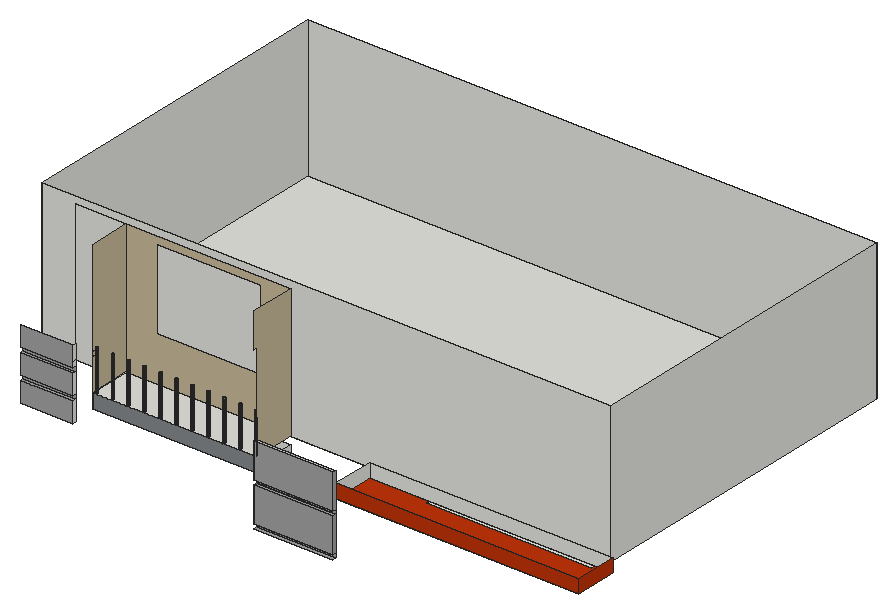
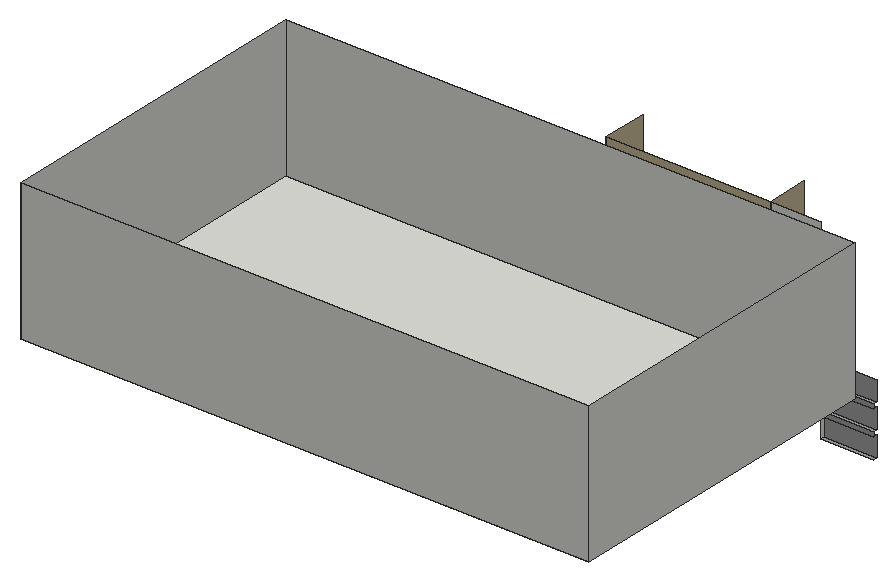
# SketchUp Ruby script. Lengths in inches.
U = 1.inch
M = Sketchup.active_model
def pt(a) = Geom::Point3d.new(a.map { |v| v * U })
def face(e, loops, mat)
  f = e.add_face(loops[0].map { |a| pt(a) })
  loops[1..].each { |l| e.add_face(l.map { |a| pt(a) }).erase! }
  f.material = f.back_material = mat if mat
  f
end
# faces: each face lists its corners as indices into pts; further lists are holes
def faces(e, pts, list, mat = nil) = list.each { |f| face(e, (f[0].is_a?(Array) ? f : [f]).map { |l| l.map { |i| pts[i] } }, mat) }
# xy, xz, yz: faces in a plane at the given z, y or x. An outline is a flat list of corners, or four numbers for a rectangle; further outlines are holes
def ring(l) = l.size == 4 ? [[l[0], l[1]], [l[2], l[1]], [l[2], l[3]], [l[0], l[3]]] : l.each_slice(2).to_a
def flat(e, list, mat, &to3) = list.each { |f| face(e, (f[0].is_a?(Array) ? f : [f]).map { |l| ring(l).map { |u, v| to3.(u, v) } }, mat) }
def xy(e, z, list, mat = nil) = flat(e, list, mat) { |x, y| [x, y, z] }
def xz(e, y, list, mat = nil) = flat(e, list, mat) { |x, z| [x, y, z] }
def yz(e, x, list, mat = nil) = flat(e, list, mat) { |y, z| [x, y, z] }
def lines(e, pts, list) = list.each { |a, b| e.add_line(pt(pts[a]), pt(pts[b])) }
# prism: a flat outline (further loops are holes) pulled along v
def prism(e, loops, v, mat = nil)
  f = face(e, loops, mat); d = Geom::Vector3d.new(v.map { |x| x * U })
  f.pushpull(f.normal.samedirection?(d) ? d.length : -d.length)
end
def box(e, o, s, mat = nil) = prism(e, [[o, [o[0] + s[0], o[1], o[2]], [o[0] + s[0], o[1] + s[1], o[2]], [o[0], o[1] + s[1], o[2]]]], [0, 0, s[2]], mat)
def at(x, y, z, deg = 0) = Geom::Transformation.translation(pt([x, y, z])) * Geom::Transformation.rotation(ORIGIN, Z_AXIS, deg.degrees)
def axes(o, x, y, z) = Geom::Transformation.new([*x, 0, *y, 0, *z, 0, *pt(o).to_a, 1])
def part(name) = M.definitions.add(name)
# library, detail: a bought-in or finely detailed component or shape, given as its bounding box
def library(name, o, s) = part(name).tap { |d| box(d.entities, o, s) }
def detail(e, o, s) = box(e.add_group.entities, o, s)
def put(e, d, t, mat = nil) = e.add_instance(d, t).tap { |i| i.material = mat if mat }
def group(e, t, mat = nil) = e.add_group.tap { |g| g.transformation = t; g.material = mat if mat }.entities
root = M.entities
M.materials.add("[0133_Gray]").color = [128, 128, 128]
M.materials.add("[Blacktop New]").color = [30, 30, 30]
M.materials.add("[Blacktop Old 01]").color = [132, 136, 139]
M.materials.add("[Marble Carrara Gold Floor Tile]").color = [225, 223, 217]
M.materials.add("[Modern Siding]1").color = [191, 52, 9]
M.materials.add("[Pavers Flagstone Gray]").color = [162, 162, 162]
M.materials.add("[Quartz Light Brown]").color = [199, 184, 152]
xy(root,432.5,[[229.62,0,297.58,3]],"[Pavers Flagstone Gray]")
xy(root,432.57,[[0,36,45.0625,39]],"[Pavers Flagstone Gray]")
xy(root,436.12,[[229.62,0,297.58,3]],"[Pavers Flagstone Gray]")
xy(root,449.9375,[[0,36,45.0625,39]],"[Pavers Flagstone Gray]")
xy(root,454.01,[[0,36,45.0625,39]],"[Pavers Flagstone Gray]")
xy(root,464.74,[[127.42,36,161.55,39],[163.99,36,195.67,39]],"[Blacktop New]")
xy(root,466,[[229.62,0,297.58,3]],"[Pavers Flagstone Gray]")
xy(root,467.74,[[124.42,36,198.67,39]],"[Blacktop New]")
xy(root,469.62,[[229.62,0,297.58,3]],"[Pavers Flagstone Gray]")
xy(root,471.375,[[0,36,45.0625,39]],"[Pavers Flagstone Gray]")
xy(root,472.125,[[355.33,36,420.06,39],[424.01,36,484.79,39]],"[Blacktop New]")
xy(root,473.6875,[[88.53,3,229.62,39]],"[Blacktop Old 01]")
xy(root,475.45,[[0,36,45.0625,39]],"[Pavers Flagstone Gray]")
xy(root,478.125,[[349.33,36,490.79,39]])
xy(root,478.125,[[297.58,3,297.58,39,349.33,39,349.33,36,490.79,36,490.79,39,506.625,39,506.625,3]],"[Modern Siding]1")
xy(root,480,[[9,48,497.625,333.4375]])
xy(root,486.23,[[[88.53,3,229.62,39],[104.73,3.35,104.5,3.39,104.3,3.49,104.13,3.65,104,3.84,103.93,4.05,103.92,4.28,103.97,4.51,104.07,4.71,104.22,4.88,104.41,5.01,104.63,5.08,104.86,5.09,105.08,5.04,105.28,4.94,105.45,4.79,105.58,4.6,105.65,4.38,105.66,4.15,105.62,3.93,105.51,3.73,105.36,3.55,105.17,3.43,104.95,3.36],[118.41,3.35,118.19,3.39,117.99,3.49,117.82,3.65,117.69,3.84,117.62,4.05,117.61,4.28,117.65,4.51,117.76,4.71,117.91,4.88,118.1,5.01,118.32,5.08,118.54,5.09,118.77,5.04,118.97,4.94,119.14,4.79,119.27,4.6,119.34,4.38,119.35,4.15,119.31,3.93,119.2,3.73,119.05,3.55,118.86,3.43,118.64,3.36],[132.1,3.35,131.88,3.39,131.67,3.49,131.5,3.65,131.38,3.84,131.31,4.05,131.29,4.28,131.34,4.51,131.44,4.71,131.6,4.88,131.79,5.01,132,5.08,132.23,5.09,132.46,5.04,132.66,4.94,132.83,4.79,132.95,4.6,133.03,4.38,133.04,4.15,132.99,3.93,132.89,3.73,132.74,3.55,132.55,3.43,132.33,3.36],[145.79,3.35,145.57,3.39,145.36,3.49,145.19,3.65,145.07,3.84,144.99,4.05,144.98,4.28,145.03,4.51,145.13,4.71,145.28,4.88,145.47,5.01,145.69,5.08,145.92,5.09,146.14,5.04,146.35,4.94,146.52,4.79,146.64,4.6,146.71,4.38,146.73,4.15,146.68,3.93,146.58,3.73,146.43,3.55,146.23,3.43,146.02,3.36],[159.48,3.35,159.25,3.39,159.05,3.49,158.88,3.65,158.75,3.84,158.68,4.05,158.67,4.28,158.72,4.51,158.82,4.71,158.97,4.88,159.16,5.01,159.38,5.08,159.61,5.09,159.83,5.04,160.03,4.94,160.2,4.79,160.33,4.6,160.4,4.38,160.41,4.15,160.37,3.93,160.26,3.73,160.11,3.55,159.92,3.43,159.7,3.36],[173.16,3.35,172.94,3.39,172.74,3.49,172.57,3.65,172.44,3.84,172.37,4.05,172.36,4.28,172.4,4.51,172.51,4.71,172.66,4.88,172.85,5.01,173.07,5.08,173.29,5.09,173.52,5.04,173.72,4.94,173.89,4.79,174.02,4.6,174.09,4.38,174.1,4.15,174.06,3.93,173.95,3.73,173.8,3.55,173.61,3.43,173.39,3.36],[91.04,3.35,90.82,3.39,90.61,3.49,90.44,3.65,90.32,3.84,90.24,4.05,90.23,4.28,90.28,4.51,90.38,4.71,90.53,4.88,90.72,5.01,90.94,5.08,91.17,5.09,91.39,5.04,91.6,4.94,91.77,4.79,91.89,4.6,91.96,4.38,91.98,4.15,91.93,3.93,91.83,3.73,91.68,3.55,91.48,3.43,91.27,3.36],[186.85,3.35,186.63,3.39,186.42,3.49,186.25,3.65,186.13,3.84,186.06,4.05,186.04,4.28,186.09,4.51,186.19,4.71,186.35,4.88,186.54,5.01,186.75,5.08,186.98,5.09,187.21,5.04,187.41,4.94,187.58,4.79,187.7,4.6,187.78,4.38,187.79,4.15,187.74,3.93,187.64,3.73,187.49,3.55,187.3,3.43,187.08,3.36],[200.54,3.35,200.32,3.39,200.11,3.49,199.94,3.65,199.82,3.84,199.74,4.05,199.73,4.28,199.78,4.51,199.88,4.71,200.03,4.88,200.22,5.01,200.44,5.08,200.67,5.09,200.89,5.04,201.1,4.94,201.27,4.79,201.39,4.6,201.46,4.38,201.48,4.15,201.43,3.93,201.33,3.73,201.18,3.55,200.98,3.43,200.77,3.36],[214.23,3.35,214,3.39,213.8,3.49,213.63,3.65,213.5,3.84,213.43,4.05,213.42,4.28,213.47,4.51,213.57,4.71,213.72,4.88,213.91,5.01,214.13,5.08,214.36,5.09,214.58,5.04,214.78,4.94,214.95,4.79,215.08,4.6,215.15,4.38,215.16,4.15,215.12,3.93,215.01,3.73,214.86,3.55,214.67,3.43,214.45,3.36],[227.91,3.35,227.69,3.39,227.49,3.49,227.32,3.65,227.19,3.84,227.12,4.05,227.11,4.28,227.15,4.51,227.26,4.71,227.41,4.88,227.6,5.01,227.82,5.08,228.04,5.09,228.27,5.04,228.47,4.94,228.64,4.79,228.77,4.6,228.84,4.38,228.85,4.15,228.81,3.93,228.7,3.73,228.55,3.55,228.36,3.43,228.14,3.36]]],"[Marble Carrara Gold Floor Tile]")
xz(root,0,[[229.62,436.12,297.58,466],[229.62,469.62,297.58,499.5]],"[Pavers Flagstone Gray]")
xz(root,3,[[229.62,436.12,297.58,466],[229.62,469.62,297.58,499.5]])
xz(root,3,[[88.53,473.6875,229.62,486.23]],"[Blacktop Old 01]")
xz(root,3,[[297.58,478.125,506.625,489.7]],"[Modern Siding]1")
xz(root,3,[[229.62,432.5,297.58,436.12],[229.62,466,297.58,469.62]],"[Pavers Flagstone Gray]")
xz(root,36,[[0,432.57,45.0625,449.9375],[0,454.01,45.0625,471.375],[0,475.45,45.0625,492.8125]],"[Pavers Flagstone Gray]")
xz(root,39,[[88.53,473.6875,229.62,480],[297.58,478.125,506.625,489.7],[45.0625,480,88.53,600]])
xz(root,39,[[0,449.9375,45.0625,454.01],[0,471.375,45.0625,475.45]],"[Pavers Flagstone Gray]")
xz(root,39,[[[88.53,486.23,229.62,600],[114.78,524.95,204.16,593.82]]],"[Quartz Light Brown]")
xz(root,48,[[9,480,497.625,600]])
xz(root,333.4375,[[9,480,497.625,600]])
yz(root,9,[[48,480,333.4375,600]])
yz(root,45.0625,[[36,432.57,39,449.9375],[36,454.01,39,471.375],[36,475.45,39,480],[36,480,39,492.8125]])
yz(root,88.53,[[3,473.6875,39,480],[3,480,39,486.23]])
yz(root,88.53,[[[3,486.23,39,600],[4.3,513.17,4.09,513.19,3.9,513.27,3.73,513.4,3.6,513.57,3.52,513.77,3.49,513.98,3.52,514.1875,3.6,514.38,3.73,514.55,3.9,514.68,4.09,514.76,4.3,514.79,4.51,514.76,4.71,514.68,4.88,514.55,5.01,514.38,5.09,514.1875,5.12,513.98,5.09,513.77,5.01,513.57,4.88,513.4,4.71,513.27,4.51,513.19],[4.3,516.98,4.09,517.01,3.9,517.09,3.73,517.22,3.6,517.38,3.52,517.58,3.49,517.79,3.52,518,3.6,518.2,3.73,518.36,3.9,518.49,4.09,518.58,4.3,518.6,4.51,518.58,4.71,518.49,4.88,518.36,5.01,518.2,5.09,518,5.12,517.79,5.09,517.58,5.01,517.38,4.88,517.22,4.71,517.09,4.51,517.01],[4.3,490.29,4.09,490.32,3.9,490.4,3.73,490.53,3.6,490.7,3.52,490.89,3.49,491.1,3.52,491.3125,3.6,491.51,3.73,491.68,3.9,491.81,4.09,491.89,4.3,491.92,4.51,491.89,4.71,491.81,4.88,491.68,5.01,491.51,5.09,491.3125,5.12,491.1,5.09,490.89,5.01,490.7,4.88,490.53,4.71,490.4,4.51,490.32],[4.3,494.1,4.09,494.13,3.9,494.21,3.73,494.34,3.6,494.51,3.52,494.71,3.49,494.92,3.52,495.125,3.6,495.32,3.73,495.49,3.9,495.62,4.09,495.7,4.3,495.73,4.51,495.7,4.71,495.62,4.88,495.49,5.01,495.32,5.09,495.125,5.12,494.92,5.09,494.71,5.01,494.51,4.88,494.34,4.71,494.21,4.51,494.13],[4.3,497.92,4.09,497.94,3.9,498.02,3.73,498.15,3.6,498.32,3.52,498.52,3.49,498.73,3.52,498.9375,3.6,499.13,3.73,499.3,3.9,499.43,4.09,499.51,4.3,499.54,4.51,499.51,4.71,499.43,4.88,499.3,5.01,499.13,5.09,498.9375,5.12,498.73,5.09,498.52,5.01,498.32,4.88,498.15,4.71,498.02,4.51,497.94],[4.3,501.73,4.09,501.76,3.9,501.84,3.73,501.97,3.6,502.13,3.52,502.33,3.49,502.54,3.52,502.75,3.6,502.95,3.73,503.11,3.9,503.24,4.09,503.33,4.3,503.35,4.51,503.33,4.71,503.24,4.88,503.11,5.01,502.95,5.09,502.75,5.12,502.54,5.09,502.33,5.01,502.13,4.88,501.97,4.71,501.84,4.51,501.76],[4.3,505.54,4.09,505.57,3.9,505.65,3.73,505.78,3.6,505.95,3.52,506.14,3.49,506.35,3.52,506.5625,3.6,506.76,3.73,506.93,3.9,507.06,4.09,507.14,4.3,507.17,4.51,507.14,4.71,507.06,4.88,506.93,5.01,506.76,5.09,506.5625,5.12,506.35,5.09,506.14,5.01,505.95,4.88,505.78,4.71,505.65,4.51,505.57],[4.3,509.35,4.09,509.38,3.9,509.46,3.73,509.59,3.6,509.76,3.52,509.96,3.49,510.17,3.52,510.375,3.6,510.57,3.73,510.74,3.9,510.87,4.09,510.95,4.3,510.98,4.51,510.95,4.71,510.87,4.88,510.74,5.01,510.57,5.09,510.375,5.12,510.17,5.09,509.96,5.01,509.76,4.88,509.59,4.71,509.46,4.51,509.38]]],"[Quartz Light Brown]")
yz(root,229.62,[[3,473.6875,39,480]])
yz(root,229.62,[[0,436.12,3,466],[0,469.62,3,499.5]],"[Pavers Flagstone Gray]")
yz(root,229.62,[[[3,486.23,3,570.12,0,570.12,0,600,39,600,39,486.23],[4.3,516.98,4.51,517.01,4.71,517.09,4.88,517.22,5.01,517.38,5.09,517.58,5.12,517.79,5.09,518,5.01,518.2,4.88,518.36,4.71,518.49,4.51,518.58,4.3,518.6,4.09,518.58,3.9,518.49,3.73,518.36,3.6,518.2,3.52,518,3.49,517.79,3.52,517.58,3.6,517.38,3.73,517.22,3.9,517.09,4.09,517.01],[4.3,513.17,4.51,513.19,4.71,513.27,4.88,513.4,5.01,513.57,5.09,513.77,5.12,513.98,5.09,514.1875,5.01,514.38,4.88,514.55,4.71,514.68,4.51,514.76,4.3,514.79,4.09,514.76,3.9,514.68,3.73,514.55,3.6,514.38,3.52,514.1875,3.49,513.98,3.52,513.77,3.6,513.57,3.73,513.4,3.9,513.27,4.09,513.19],[4.3,509.35,4.51,509.38,4.71,509.46,4.88,509.59,5.01,509.76,5.09,509.96,5.12,510.17,5.09,510.375,5.01,510.57,4.88,510.74,4.71,510.87,4.51,510.95,4.3,510.98,4.09,510.95,3.9,510.87,3.73,510.74,3.6,510.57,3.52,510.375,3.49,510.17,3.52,509.96,3.6,509.76,3.73,509.59,3.9,509.46,4.09,509.38],[4.3,505.54,4.51,505.57,4.71,505.65,4.88,505.78,5.01,505.95,5.09,506.14,5.12,506.35,5.09,506.5625,5.01,506.76,4.88,506.93,4.71,507.06,4.51,507.14,4.3,507.17,4.09,507.14,3.9,507.06,3.73,506.93,3.6,506.76,3.52,506.5625,3.49,506.35,3.52,506.14,3.6,505.95,3.73,505.78,3.9,505.65,4.09,505.57],[4.3,501.73,4.51,501.76,4.71,501.84,4.88,501.97,5.01,502.13,5.09,502.33,5.12,502.54,5.09,502.75,5.01,502.95,4.88,503.11,4.71,503.24,4.51,503.33,4.3,503.35,4.09,503.33,3.9,503.24,3.73,503.11,3.6,502.95,3.52,502.75,3.49,502.54,3.52,502.33,3.6,502.13,3.73,501.97,3.9,501.84,4.09,501.76],[4.3,490.29,4.51,490.32,4.71,490.4,4.88,490.53,5.01,490.7,5.09,490.89,5.12,491.1,5.09,491.3125,5.01,491.51,4.88,491.68,4.71,491.81,4.51,491.89,4.3,491.92,4.09,491.89,3.9,491.81,3.73,491.68,3.6,491.51,3.52,491.3125,3.49,491.1,3.52,490.89,3.6,490.7,3.73,490.53,3.9,490.4,4.09,490.32]]],"[Quartz Light Brown]")
yz(root,297.58,[[3,478.125,39,489.7]])
yz(root,297.58,[[0,436.12,3,466],[0,469.62,3,499.5]],"[Pavers Flagstone Gray]")
yz(root,497.625,[[48,480,333.4375,600]])
yz(root,506.625,[[3,478.125,39,489.7]],"[Modern Siding]1")
p = [[90.82,3.39,486.23],[91.04,3.35,486.23],[91.04,3.35,521.04],[90.82,3.39,521.04],[91.27,3.36,486.23],[91.27,3.36,521.04],
  [104.5,3.39,486.23],[104.73,3.35,486.23],[104.73,3.35,521.04],[104.5,3.39,521.04],[104.95,3.36,486.23],[104.95,3.36,521.04],
  [118.19,3.39,486.23],[118.41,3.35,486.23],[118.41,3.35,521.04],[118.19,3.39,521.04],[118.64,3.36,486.23],[118.64,3.36,521.04],
  [131.88,3.39,486.23],[132.1,3.35,486.23],[132.1,3.35,521.04],[131.88,3.39,521.04],[132.33,3.36,486.23],[132.33,3.36,521.04],
  [145.57,3.39,486.23],[145.79,3.35,486.23],[145.79,3.35,521.04],[145.57,3.39,521.04],[146.02,3.36,486.23],[146.02,3.36,521.04],
  [159.25,3.39,486.23],[159.48,3.35,486.23],[159.48,3.35,521.04],[159.25,3.39,521.04],[159.7,3.36,486.23],[159.7,3.36,521.04],
  [172.94,3.39,486.23],[173.16,3.35,486.23],[173.16,3.35,521.04],[172.94,3.39,521.04],[173.39,3.36,486.23],[173.39,3.36,521.04],
  [186.63,3.39,486.23],[186.85,3.35,486.23],[186.85,3.35,521.04],[186.63,3.39,521.04],[187.08,3.36,486.23],[187.08,3.36,521.04],
  [200.32,3.39,486.23],[200.54,3.35,486.23],[200.54,3.35,521.04],[200.32,3.39,521.04],[200.77,3.36,486.23],[200.77,3.36,521.04],
  [214,3.39,486.23],[214.23,3.35,486.23],[214.23,3.35,521.04],[214,3.39,521.04],[214.45,3.36,486.23],[214.45,3.36,521.04],
  [227.69,3.39,486.23],[227.91,3.35,486.23],[227.91,3.35,521.04],[227.69,3.39,521.04],[228.14,3.36,486.23],[228.14,3.36,521.04],
  [90.61,3.49,486.23],[90.61,3.49,521.04],[91.48,3.43,486.23],[91.48,3.43,521.04],[91.68,3.55,486.23],[91.68,3.55,521.04],
  [104.3,3.49,486.23],[104.3,3.49,521.04],[105.17,3.43,486.23],[105.17,3.43,521.04],[105.36,3.55,486.23],[105.36,3.55,521.04],
  [117.99,3.49,486.23],[117.99,3.49,521.04],[118.86,3.43,486.23],[118.86,3.43,521.04],[119.05,3.55,486.23],[119.05,3.55,521.04],
  [131.67,3.49,486.23],[131.67,3.49,521.04],[132.55,3.43,486.23],[132.55,3.43,521.04],[132.74,3.55,486.23],[132.74,3.55,521.04],
  [145.36,3.49,486.23],[145.36,3.49,521.04],[146.23,3.43,486.23],[146.23,3.43,521.04],[146.43,3.55,486.23],[146.43,3.55,521.04],
  [159.05,3.49,486.23],[159.05,3.49,521.04],[159.92,3.43,486.23],[159.92,3.43,521.04],[160.11,3.55,486.23],[160.11,3.55,521.04],
  [172.74,3.49,486.23],[172.74,3.49,521.04],[173.61,3.43,486.23],[173.61,3.43,521.04],[173.8,3.55,486.23],[173.8,3.55,521.04],
  [186.42,3.49,486.23],[186.42,3.49,521.04],[187.3,3.43,486.23],[187.3,3.43,521.04],[187.49,3.55,486.23],[187.49,3.55,521.04],
  [200.11,3.49,486.23],[200.11,3.49,521.04],[200.98,3.43,486.23],[200.98,3.43,521.04],[201.18,3.55,486.23],[201.18,3.55,521.04],
  [213.8,3.49,486.23],[213.8,3.49,521.04],[214.67,3.43,486.23],[214.67,3.43,521.04],[214.86,3.55,486.23],[214.86,3.55,521.04],
  [227.49,3.49,486.23],[227.49,3.49,521.04],[228.36,3.43,486.23],[228.36,3.43,521.04],[228.55,3.55,486.23],[228.55,3.55,521.04],
  [90.44,3.65,486.23],[90.44,3.65,521.04],[104.13,3.65,486.23],[104.13,3.65,521.04],[117.82,3.65,486.23],[117.82,3.65,521.04],
  [131.5,3.65,486.23],[131.5,3.65,521.04],[145.19,3.65,486.23],[145.19,3.65,521.04],[158.88,3.65,486.23],[158.88,3.65,521.04],
  [172.57,3.65,486.23],[172.57,3.65,521.04],[186.25,3.65,486.23],[186.25,3.65,521.04],[199.94,3.65,486.23],[199.94,3.65,521.04],
  [213.63,3.65,486.23],[213.63,3.65,521.04],[227.32,3.65,486.23],[227.32,3.65,521.04],[90.32,3.84,486.23],[90.32,3.84,521.04],
  [91.83,3.73,486.23],[91.83,3.73,521.04],[104,3.84,486.23],[104,3.84,521.04],[105.51,3.73,486.23],[105.51,3.73,521.04],
  [117.69,3.84,486.23],[117.69,3.84,521.04],[119.2,3.73,486.23],[119.2,3.73,521.04],[131.38,3.84,486.23],[131.38,3.84,521.04],
  [132.89,3.73,486.23],[132.89,3.73,521.04],[145.07,3.84,486.23],[145.07,3.84,521.04],[146.58,3.73,486.23],[146.58,3.73,521.04],
  [158.75,3.84,486.23],[158.75,3.84,521.04],[160.26,3.73,486.23],[160.26,3.73,521.04],[172.44,3.84,486.23],[172.44,3.84,521.04],
  [173.95,3.73,486.23],[173.95,3.73,521.04],[186.13,3.84,486.23],[186.13,3.84,521.04],[187.64,3.73,486.23],[187.64,3.73,521.04],
  [199.82,3.84,486.23],[199.82,3.84,521.04],[201.33,3.73,486.23],[201.33,3.73,521.04],[213.5,3.84,486.23],[213.5,3.84,521.04],
  [215.01,3.73,486.23],[215.01,3.73,521.04],[227.19,3.84,486.23],[227.19,3.84,521.04],[228.7,3.73,486.23],[228.7,3.73,521.04],
  [91.93,3.93,486.23],[91.93,3.93,521.04],[105.62,3.93,486.23],[105.62,3.93,521.04],[119.31,3.93,486.23],[119.31,3.93,521.04],
  [132.99,3.93,486.23],[132.99,3.93,521.04],[146.68,3.93,486.23],[146.68,3.93,521.04],[160.37,3.93,486.23],[160.37,3.93,521.04],
  [174.06,3.93,486.23],[174.06,3.93,521.04],[187.74,3.93,486.23],[187.74,3.93,521.04],[201.43,3.93,486.23],[201.43,3.93,521.04],
  [215.12,3.93,486.23],[215.12,3.93,521.04],[228.81,3.93,486.23],[228.81,3.93,521.04],[90.24,4.05,486.23],[90.24,4.05,521.04],
  [103.93,4.05,486.23],[103.93,4.05,521.04],[117.62,4.05,486.23],[117.62,4.05,521.04],[131.31,4.05,486.23],[131.31,4.05,521.04],
  [144.99,4.05,486.23],[144.99,4.05,521.04],[158.68,4.05,486.23],[158.68,4.05,521.04],[172.37,4.05,486.23],[172.37,4.05,521.04],
  [186.06,4.05,486.23],[186.06,4.05,521.04],[199.74,4.05,486.23],[199.74,4.05,521.04],[213.43,4.05,486.23],[213.43,4.05,521.04],
  [227.12,4.05,486.23],[227.12,4.05,521.04],[91.98,4.15,486.23],[91.98,4.15,521.04],[105.66,4.15,486.23],[105.66,4.15,521.04],
  [119.35,4.15,486.23],[119.35,4.15,521.04],[133.04,4.15,486.23],[133.04,4.15,521.04],[146.73,4.15,486.23],[146.73,4.15,521.04],
  [160.41,4.15,486.23],[160.41,4.15,521.04],[174.1,4.15,486.23],[174.1,4.15,521.04],[187.79,4.15,486.23],[187.79,4.15,521.04],
  [201.48,4.15,486.23],[201.48,4.15,521.04],[215.16,4.15,486.23],[215.16,4.15,521.04],[228.85,4.15,486.23],[228.85,4.15,521.04],
  [90.23,4.28,486.23],[90.23,4.28,521.04],[103.92,4.28,486.23],[103.92,4.28,521.04],[117.61,4.28,486.23],[117.61,4.28,521.04],
  [131.29,4.28,486.23],[131.29,4.28,521.04],[144.98,4.28,486.23],[144.98,4.28,521.04],[158.67,4.28,486.23],[158.67,4.28,521.04],
  [172.36,4.28,486.23],[172.36,4.28,521.04],[186.04,4.28,486.23],[186.04,4.28,521.04],[199.73,4.28,486.23],[199.73,4.28,521.04],
  [213.42,4.28,486.23],[213.42,4.28,521.04],[227.11,4.28,486.23],[227.11,4.28,521.04],[91.96,4.38,486.23],[91.96,4.38,521.04],
  [105.65,4.38,486.23],[105.65,4.38,521.04],[119.34,4.38,486.23],[119.34,4.38,521.04],[133.03,4.38,486.23],[133.03,4.38,521.04],
  [146.71,4.38,486.23],[146.71,4.38,521.04],[160.4,4.38,486.23],[160.4,4.38,521.04],[174.09,4.38,486.23],[174.09,4.38,521.04],
  [187.78,4.38,486.23],[187.78,4.38,521.04],[201.46,4.38,486.23],[201.46,4.38,521.04],[215.15,4.38,486.23],[215.15,4.38,521.04],
  [228.84,4.38,486.23],[228.84,4.38,521.04],[90.28,4.51,486.23],[90.28,4.51,521.04],[103.97,4.51,486.23],[103.97,4.51,521.04],
  [117.65,4.51,486.23],[117.65,4.51,521.04],[131.34,4.51,486.23],[131.34,4.51,521.04],[145.03,4.51,486.23],[145.03,4.51,521.04],
  [158.72,4.51,486.23],[158.72,4.51,521.04],[172.4,4.51,486.23],[172.4,4.51,521.04],[186.09,4.51,486.23],[186.09,4.51,521.04],
  [199.78,4.51,486.23],[199.78,4.51,521.04],[213.47,4.51,486.23],[213.47,4.51,521.04],[227.15,4.51,486.23],[227.15,4.51,521.04],
  [91.89,4.6,486.23],[91.89,4.6,521.04],[105.58,4.6,486.23],[105.58,4.6,521.04],[119.27,4.6,486.23],[119.27,4.6,521.04],
  [132.95,4.6,486.23],[132.95,4.6,521.04],[146.64,4.6,486.23],[146.64,4.6,521.04],[160.33,4.6,486.23],[160.33,4.6,521.04],
  [174.02,4.6,486.23],[174.02,4.6,521.04],[187.7,4.6,486.23],[187.7,4.6,521.04],[201.39,4.6,486.23],[201.39,4.6,521.04],
  [215.08,4.6,486.23],[215.08,4.6,521.04],[228.77,4.6,486.23],[228.77,4.6,521.04],[90.38,4.71,486.23],[90.38,4.71,521.04],
  [104.07,4.71,486.23],[104.07,4.71,521.04],[117.76,4.71,486.23],[117.76,4.71,521.04],[131.44,4.71,486.23],[131.44,4.71,521.04],
  [145.13,4.71,486.23],[145.13,4.71,521.04],[158.82,4.71,486.23],[158.82,4.71,521.04],[172.51,4.71,486.23],[172.51,4.71,521.04],
  [186.19,4.71,486.23],[186.19,4.71,521.04],[199.88,4.71,486.23],[199.88,4.71,521.04],[213.57,4.71,486.23],[213.57,4.71,521.04],
  [227.26,4.71,486.23],[227.26,4.71,521.04],[91.77,4.79,486.23],[91.77,4.79,521.04],[105.45,4.79,486.23],[105.45,4.79,521.04],
  [119.14,4.79,486.23],[119.14,4.79,521.04],[132.83,4.79,486.23],[132.83,4.79,521.04],[146.52,4.79,486.23],[146.52,4.79,521.04],
  [160.2,4.79,486.23],[160.2,4.79,521.04],[173.89,4.79,486.23],[173.89,4.79,521.04],[187.58,4.79,486.23],[187.58,4.79,521.04],
  [201.27,4.79,486.23],[201.27,4.79,521.04],[214.95,4.79,486.23],[214.95,4.79,521.04],[228.64,4.79,486.23],[228.64,4.79,521.04],
  [90.53,4.88,486.23],[90.53,4.88,521.04],[104.22,4.88,486.23],[104.22,4.88,521.04],[117.91,4.88,486.23],[117.91,4.88,521.04],
  [131.6,4.88,486.23],[131.6,4.88,521.04],[145.28,4.88,486.23],[145.28,4.88,521.04],[158.97,4.88,486.23],[158.97,4.88,521.04],
  [172.66,4.88,486.23],[172.66,4.88,521.04],[186.35,4.88,486.23],[186.35,4.88,521.04],[200.03,4.88,486.23],[200.03,4.88,521.04],
  [213.72,4.88,486.23],[213.72,4.88,521.04],[227.41,4.88,486.23],[227.41,4.88,521.04],[91.6,4.94,486.23],[91.6,4.94,521.04],
  [105.28,4.94,486.23],[105.28,4.94,521.04],[118.97,4.94,486.23],[118.97,4.94,521.04],[132.66,4.94,486.23],[132.66,4.94,521.04],
  [146.35,4.94,486.23],[146.35,4.94,521.04],[160.03,4.94,486.23],[160.03,4.94,521.04],[173.72,4.94,486.23],[173.72,4.94,521.04],
  [187.41,4.94,486.23],[187.41,4.94,521.04],[201.1,4.94,486.23],[201.1,4.94,521.04],[214.78,4.94,486.23],[214.78,4.94,521.04],
  [228.47,4.94,486.23],[228.47,4.94,521.04],[90.72,5.01,486.23],[90.72,5.01,521.04],[90.72,5.01,518.2],[90.72,5.01,517.38],
  [90.72,5.01,514.38],[90.72,5.01,513.57],[90.72,5.01,510.57],[90.72,5.01,509.76],[90.72,5.01,506.76],[90.72,5.01,505.95],
  [90.72,5.01,502.95],[90.72,5.01,502.13],[90.72,5.01,499.13],[90.72,5.01,498.32],[90.72,5.01,495.32],[90.72,5.01,494.51],
  [90.72,5.01,491.51],[90.72,5.01,490.7],[91.39,5.04,486.23],[91.39,5.04,521.04],[104.41,5.01,486.23],[104.41,5.01,521.04],
  [104.41,5.01,518.2],[104.41,5.01,517.38],[104.41,5.01,514.38],[104.41,5.01,513.57],[104.41,5.01,510.57],[104.41,5.01,509.76],
  [104.41,5.01,506.76],[104.41,5.01,505.95],[104.41,5.01,502.95],[104.41,5.01,502.13],[104.41,5.01,499.13],[104.41,5.01,498.32],
  [104.41,5.01,495.32],[104.41,5.01,494.51],[104.41,5.01,491.51],[104.41,5.01,490.7],[105.08,5.04,486.23],[105.08,5.04,521.04],
  [118.1,5.01,486.23],[118.1,5.01,521.04],[118.1,5.01,518.2],[118.1,5.01,517.38],[118.1,5.01,514.38],[118.1,5.01,513.57],
  [118.1,5.01,510.57],[118.1,5.01,509.76],[118.1,5.01,506.76],[118.1,5.01,505.95],[118.1,5.01,502.95],[118.1,5.01,502.13],
  [118.1,5.01,499.13],[118.1,5.01,498.32],[118.1,5.01,495.32],[118.1,5.01,494.51],[118.1,5.01,491.51],[118.1,5.01,490.7],
  [118.77,5.04,486.23],[118.77,5.04,521.04],[131.79,5.01,486.23],[131.79,5.01,521.04],[131.79,5.01,518.2],[131.79,5.01,517.38],
  [131.79,5.01,514.38],[131.79,5.01,513.57],[131.79,5.01,510.57],[131.79,5.01,509.76],[131.79,5.01,506.76],[131.79,5.01,505.95],
  [131.79,5.01,502.95],[131.79,5.01,502.13],[131.79,5.01,499.13],[131.79,5.01,498.32],[131.79,5.01,495.32],[131.79,5.01,494.51],
  [131.79,5.01,491.51],[131.79,5.01,490.7],[132.46,5.04,486.23],[132.46,5.04,521.04],[145.47,5.01,486.23],[145.47,5.01,521.04],
  [145.47,5.01,518.2],[145.47,5.01,517.38],[145.47,5.01,514.38],[145.47,5.01,513.57],[145.47,5.01,510.57],[145.47,5.01,509.76],
  [145.47,5.01,506.76],[145.47,5.01,505.95],[145.47,5.01,502.95],[145.47,5.01,502.13],[145.47,5.01,499.13],[145.47,5.01,498.32],
  [145.47,5.01,495.32],[145.47,5.01,494.51],[145.47,5.01,491.51],[145.47,5.01,490.7],[146.14,5.04,486.23],[146.14,5.04,521.04],
  [159.16,5.01,486.23],[159.16,5.01,521.04],[159.16,5.01,518.2],[159.16,5.01,517.38],[159.16,5.01,514.38],[159.16,5.01,513.57],
  [159.16,5.01,510.57],[159.16,5.01,509.76],[159.16,5.01,506.76],[159.16,5.01,505.95],[159.16,5.01,502.95],[159.16,5.01,502.13],
  [159.16,5.01,499.13],[159.16,5.01,498.32],[159.16,5.01,495.32],[159.16,5.01,494.51],[159.16,5.01,491.51],[159.16,5.01,490.7],
  [159.83,5.04,486.23],[159.83,5.04,521.04],[172.85,5.01,486.23],[172.85,5.01,521.04],[172.85,5.01,518.2],[172.85,5.01,517.38],
  [172.85,5.01,514.38],[172.85,5.01,513.57],[172.85,5.01,510.57],[172.85,5.01,509.76],[172.85,5.01,506.76],[172.85,5.01,505.95],
  [172.85,5.01,502.95],[172.85,5.01,502.13],[172.85,5.01,499.13],[172.85,5.01,498.32],[172.85,5.01,495.32],[172.85,5.01,494.51],
  [172.85,5.01,491.51],[172.85,5.01,490.7],[173.52,5.04,486.23],[173.52,5.04,521.04],[186.54,5.01,486.23],[186.54,5.01,521.04],
  [186.54,5.01,518.2],[186.54,5.01,517.38],[186.54,5.01,514.38],[186.54,5.01,513.57],[186.54,5.01,510.57],[186.54,5.01,509.76],
  [186.54,5.01,506.76],[186.54,5.01,505.95],[186.54,5.01,502.95],[186.54,5.01,502.13],[186.54,5.01,499.13],[186.54,5.01,498.32],
  [186.54,5.01,495.32],[186.54,5.01,494.51],[186.54,5.01,491.51],[186.54,5.01,490.7],[187.21,5.04,486.23],[187.21,5.04,521.04],
  [200.22,5.01,486.23],[200.22,5.01,521.04],[200.22,5.01,518.2],[200.22,5.01,517.38],[200.22,5.01,514.38],[200.22,5.01,513.57],
  [200.22,5.01,510.57],[200.22,5.01,509.76],[200.22,5.01,506.76],[200.22,5.01,505.95],[200.22,5.01,502.95],[200.22,5.01,502.13],
  [200.22,5.01,499.13],[200.22,5.01,498.32],[200.22,5.01,495.32],[200.22,5.01,494.51],[200.22,5.01,491.51],[200.22,5.01,490.7],
  [200.89,5.04,486.23],[200.89,5.04,521.04],[213.91,5.01,486.23],[213.91,5.01,521.04],[213.91,5.01,518.2],[213.91,5.01,517.38],
  [213.91,5.01,514.38],[213.91,5.01,513.57],[213.91,5.01,510.57],[213.91,5.01,509.76],[213.91,5.01,506.76],[213.91,5.01,505.95],
  [213.91,5.01,502.95],[213.91,5.01,502.13],[213.91,5.01,499.13],[213.91,5.01,498.32],[213.91,5.01,495.32],[213.91,5.01,494.51],
  [213.91,5.01,491.51],[213.91,5.01,490.7],[214.58,5.04,486.23],[214.58,5.04,521.04],[227.6,5.01,486.23],[227.6,5.01,521.04],
  [227.6,5.01,518.2],[227.6,5.01,517.38],[227.6,5.01,514.38],[227.6,5.01,513.57],[227.6,5.01,510.57],[227.6,5.01,509.76],
  [227.6,5.01,506.76],[227.6,5.01,505.95],[227.6,5.01,502.95],[227.6,5.01,502.13],[227.6,5.01,499.13],[227.6,5.01,498.32],
  [227.6,5.01,495.32],[227.6,5.01,494.51],[227.6,5.01,491.51],[227.6,5.01,490.7],[228.27,5.04,486.23],[228.27,5.04,521.04],
  [90.94,5.08,486.23],[90.94,5.08,521.04],[91.17,5.09,486.23],[91.17,5.09,521.04],[104.63,5.08,486.23],[104.63,5.08,521.04],
  [104.86,5.09,486.23],[104.86,5.09,521.04],[118.32,5.08,486.23],[118.32,5.08,521.04],[118.54,5.09,486.23],[118.54,5.09,521.04],
  [132,5.08,486.23],[132,5.08,521.04],[132.23,5.09,486.23],[132.23,5.09,521.04],[145.69,5.08,486.23],[145.69,5.08,521.04],
  [145.92,5.09,486.23],[145.92,5.09,521.04],[159.38,5.08,486.23],[159.38,5.08,521.04],[159.61,5.09,486.23],[159.61,5.09,521.04],
  [173.07,5.08,486.23],[173.07,5.08,521.04],[173.29,5.09,486.23],[173.29,5.09,521.04],[186.75,5.08,486.23],[186.75,5.08,521.04],
  [186.98,5.09,486.23],[186.98,5.09,521.04],[200.44,5.08,486.23],[200.44,5.08,521.04],[200.67,5.09,486.23],[200.67,5.09,521.04],
  [214.13,5.08,486.23],[214.13,5.08,521.04],[214.36,5.09,486.23],[214.36,5.09,521.04],[227.82,5.08,486.23],[227.82,5.08,521.04],
  [228.04,5.09,486.23],[228.04,5.09,521.04]]
faces(root,p,[[0,1,2,3],[1,4,5,2],[6,7,8,9],[7,10,11,8],[12,13,14,15],[13,16,17,14],[18,19,20,21],[19,22,23,20],
  [24,25,26,27],[25,28,29,26],[30,31,32,33],[31,34,35,32],[36,37,38,39],[37,40,41,38],[42,43,44,45],[43,46,47,44],
  [48,49,50,51],[49,52,53,50],[54,55,56,57],[55,58,59,56],[60,61,62,63],[61,64,65,62],[66,0,3,67],[4,68,69,5],
  [68,70,71,69],[72,6,9,73],[10,74,75,11],[74,76,77,75],[78,12,15,79],[16,80,81,17],[80,82,83,81],[84,18,21,85],
  [22,86,87,23],[86,88,89,87],[90,24,27,91],[28,92,93,29],[92,94,95,93],[96,30,33,97],[34,98,99,35],[98,100,101,99],
  [102,36,39,103],[40,104,105,41],[104,106,107,105],[108,42,45,109],[46,110,111,47],[110,112,113,111],[114,48,51,115],[52,116,117,53],
  [116,118,119,117],[120,54,57,121],[58,122,123,59],[122,124,125,123],[126,60,63,127],[64,128,129,65],[128,130,131,129],[132,66,67,133],
  [134,72,73,135],[136,78,79,137],[138,84,85,139],[140,90,91,141],[142,96,97,143],[144,102,103,145],[146,108,109,147],[148,114,115,149],
  [150,120,121,151],[152,126,127,153],[154,132,133,155],[70,156,157,71],[158,134,135,159],[76,160,161,77],[162,136,137,163],[82,164,165,83],
  [166,138,139,167],[88,168,169,89],[170,140,141,171],[94,172,173,95],[174,142,143,175],[100,176,177,101],[178,144,145,179],[106,180,181,107],
  [182,146,147,183],[112,184,185,113],[186,148,149,187],[118,188,189,119],[190,150,151,191],[124,192,193,125],[194,152,153,195],[130,196,197,131],
  [156,198,199,157],[160,200,201,161],[164,202,203,165],[168,204,205,169],[172,206,207,173],[176,208,209,177],[180,210,211,181],[184,212,213,185],
  [188,214,215,189],[192,216,217,193],[196,218,219,197],[220,154,155,221],[222,158,159,223],[224,162,163,225],[226,166,167,227],[228,170,171,229],
  [230,174,175,231],[232,178,179,233],[234,182,183,235],[236,186,187,237],[238,190,191,239],[240,194,195,241],[198,242,243,199],[200,244,245,201],
  [202,246,247,203],[204,248,249,205],[206,250,251,207],[208,252,253,209],[210,254,255,211],[212,256,257,213],[214,258,259,215],[216,260,261,217],
  [218,262,263,219],[264,220,221,265],[266,222,223,267],[268,224,225,269],[270,226,227,271],[272,228,229,273],[274,230,231,275],[276,232,233,277],
  [278,234,235,279],[280,236,237,281],[282,238,239,283],[284,240,241,285],[242,286,287,243],[244,288,289,245],[246,290,291,247],[248,292,293,249],
  [250,294,295,251],[252,296,297,253],[254,298,299,255],[256,300,301,257],[258,302,303,259],[260,304,305,261],[262,306,307,263],[308,264,265,309],
  [310,266,267,311],[312,268,269,313],[314,270,271,315],[316,272,273,317],[318,274,275,319],[320,276,277,321],[322,278,279,323],[324,280,281,325],
  [326,282,283,327],[328,284,285,329],[286,330,331,287],[288,332,333,289],[290,334,335,291],[292,336,337,293],[294,338,339,295],[296,340,341,297],
  [298,342,343,299],[300,344,345,301],[302,346,347,303],[304,348,349,305],[306,350,351,307],[352,308,309,353],[354,310,311,355],[356,312,313,357],
  [358,314,315,359],[360,316,317,361],[362,318,319,363],[364,320,321,365],[366,322,323,367],[368,324,325,369],[370,326,327,371],[372,328,329,373],
  [330,374,375,331],[332,376,377,333],[334,378,379,335],[336,380,381,337],[338,382,383,339],[340,384,385,341],[342,386,387,343],[344,388,389,345],
  [346,390,391,347],[348,392,393,349],[350,394,395,351],[396,352,353,397],[398,354,355,399],[400,356,357,401],[402,358,359,403],[404,360,361,405],
  [406,362,363,407],[408,364,365,409],[410,366,367,411],[412,368,369,413],[414,370,371,415],[416,372,373,417],[374,418,419,375],[376,420,421,377],
  [378,422,423,379],[380,424,425,381],[382,426,427,383],[384,428,429,385],[386,430,431,387],[388,432,433,389],[390,434,435,391],[392,436,437,393],
  [394,438,439,395],[440,396,397,441,442,443,444,445,446,447,448,449,450,451,452,453,454,455,456,457],[418,458,459,419],[460,398,399,461,462,463,464,465,466,467,468,469,470,471,472,473,474,475,476,477],[420,478,479,421],[480,400,401,481,482,483,484,485,486,487,488,489,490,491,492,493,494,495,496,497],[422,498,499,423],[500,402,403,501,502,503,504,505,506,507,508,509,510,511,512,513,514,515,516,517],
  [424,518,519,425],[520,404,405,521,522,523,524,525,526,527,528,529,530,531,532,533,534,535,536,537],[426,538,539,427],[540,406,407,541,542,543,544,545,546,547,548,549,550,551,552,553,554,555,556,557],[428,558,559,429],[560,408,409,561,562,563,564,565,566,567,568,569,570,571,572,573,574,575,576,577],[430,578,579,431],[580,410,411,581,582,583,584,585,586,587,588,589,590,591,592,593,594,595,596,597],
  [432,598,599,433],[600,412,413,601,602,603,604,605,606,607,608,609,610,611,612,613,614,615,616,617],[434,618,619,435],[620,414,415,621,622,623,624,625,626,627,628,629,630,631,632,633,634,635,636,637],[436,638,639,437],[640,416,417,641,642,643,644,645,646,647,648,649,650,651,652,653,654,655,656,657],[438,658,659,439],[660,440,457,456,455,454,453,452,451,450,449,448,447,446,445,444,443,442,441,661],
  [458,662,663,459],[664,460,477,476,475,474,473,472,471,470,469,468,467,466,465,464,463,462,461,665],[478,666,667,479],[668,480,497,496,495,494,493,492,491,490,489,488,487,486,485,484,483,482,481,669],[498,670,671,499],[672,500,517,516,515,514,513,512,511,510,509,508,507,506,505,504,503,502,501,673],[518,674,675,519],[676,520,537,536,535,534,533,532,531,530,529,528,527,526,525,524,523,522,521,677],
  [538,678,679,539],[680,540,557,556,555,554,553,552,551,550,549,548,547,546,545,544,543,542,541,681],[558,682,683,559],[684,560,577,576,575,574,573,572,571,570,569,568,567,566,565,564,563,562,561,685],[578,686,687,579],[688,580,597,596,595,594,593,592,591,590,589,588,587,586,585,584,583,582,581,689],[598,690,691,599],[692,600,617,616,615,614,613,612,611,610,609,608,607,606,605,604,603,602,601,693],
  [618,694,695,619],[696,620,637,636,635,634,633,632,631,630,629,628,627,626,625,624,623,622,621,697],[638,698,699,639],[700,640,657,656,655,654,653,652,651,650,649,648,647,646,645,644,643,642,641,701],[658,702,703,659],[662,660,661,663],[666,664,665,667],[670,668,669,671],
  [674,672,673,675],[678,676,677,679],[682,680,681,683],[686,684,685,687],[690,688,689,691],[694,692,693,695],[698,696,697,699],[702,700,701,703]],"[0133_Gray]")
